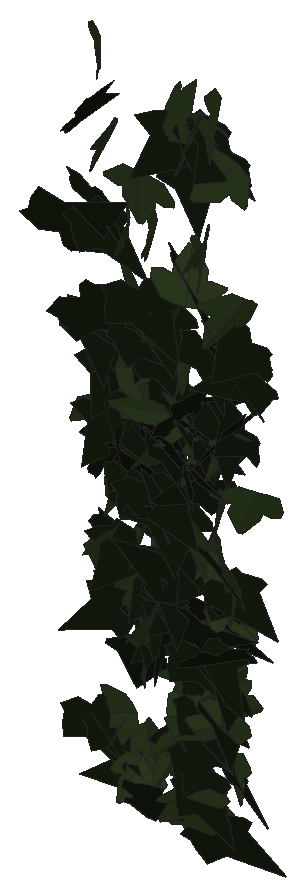
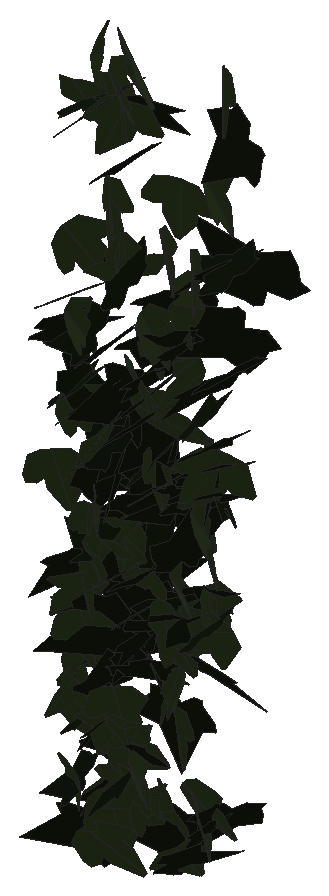
# SketchUp Ruby script. Lengths in inches.
U = 1.inch
M = Sketchup.active_model
def pt(a) = Geom::Point3d.new(a.map { |v| v * U })
def face(e, loops, mat)
  f = e.add_face(loops[0].map { |a| pt(a) })
  loops[1..].each { |l| e.add_face(l.map { |a| pt(a) }).erase! }
  f.material = f.back_material = mat if mat
  f
end
# faces: each face lists its corners as indices into pts; further lists are holes
def faces(e, pts, list, mat = nil) = list.each { |f| face(e, (f[0].is_a?(Array) ? f : [f]).map { |l| l.map { |i| pts[i] } }, mat) }
# xy, xz, yz: faces in a plane at the given z, y or x. An outline is a flat list of corners, or four numbers for a rectangle; further outlines are holes
def ring(l) = l.size == 4 ? [[l[0], l[1]], [l[2], l[1]], [l[2], l[3]], [l[0], l[3]]] : l.each_slice(2).to_a
def flat(e, list, mat, &to3) = list.each { |f| face(e, (f[0].is_a?(Array) ? f : [f]).map { |l| ring(l).map { |u, v| to3.(u, v) } }, mat) }
def xy(e, z, list, mat = nil) = flat(e, list, mat) { |x, y| [x, y, z] }
def xz(e, y, list, mat = nil) = flat(e, list, mat) { |x, z| [x, y, z] }
def yz(e, x, list, mat = nil) = flat(e, list, mat) { |y, z| [x, y, z] }
def lines(e, pts, list) = list.each { |a, b| e.add_line(pt(pts[a]), pt(pts[b])) }
# prism: a flat outline (further loops are holes) pulled along v
def prism(e, loops, v, mat = nil)
  f = face(e, loops, mat); d = Geom::Vector3d.new(v.map { |x| x * U })
  f.pushpull(f.normal.samedirection?(d) ? d.length : -d.length)
end
def box(e, o, s, mat = nil) = prism(e, [[o, [o[0] + s[0], o[1], o[2]], [o[0] + s[0], o[1] + s[1], o[2]], [o[0], o[1] + s[1], o[2]]]], [0, 0, s[2]], mat)
def at(x, y, z, deg = 0) = Geom::Transformation.translation(pt([x, y, z])) * Geom::Transformation.rotation(ORIGIN, Z_AXIS, deg.degrees)
def axes(o, x, y, z) = Geom::Transformation.new([*x, 0, *y, 0, *z, 0, *pt(o).to_a, 1])
def part(name) = M.definitions.add(name)
# library, detail: a bought-in or finely detailed component or shape, given as its bounding box
def library(name, o, s) = part(name).tap { |d| box(d.entities, o, s) }
def detail(e, o, s) = box(e.add_group.entities, o, s)
def put(e, d, t, mat = nil) = e.add_instance(d, t).tap { |i| i.material = mat if mat }
def group(e, t, mat = nil) = e.add_group.tap { |g| g.transformation = t; g.material = mat if mat }.entities
root = M.entities
M.materials.add("1026 AP 7946 SUNNY SIDE UP").color = [254, 231, 186]
M.materials.add("efeu1").color = [18, 25, 13]
M.materials.add("efeu2").color = [43, 57, 29]
c1 = part("ivyleaf_9")
p = [[1.54,2.16,1.25],[1.36,2.04,1.19],[-0.21,0.99,0.68],[-0.71,1.11,0.82],[-0.85,0.86,0.67],[-0.8,0.17,0.21],
  [-0.9,-0.01,0.1],[-0.67,-0.16,-0.02],[-0.08,-0.08,-0.05],[-0.03,-0.6,-0.4],[0.65,-0.88,-0.66],[0.83,-0.6,-0.49],
  [1.29,-0.42,-0.43],[1.8125,-0.07,-0.26],[1.21,0.44,0.15]]
faces(c1.entities,p,[[0,1,2,3,4,5,6,7,8,9,10,11,12,13,14]],"efeu1")
c2 = part("ivyleaf_10")
p = [[0,0.5,-0.03],[-0.0625,2.02,-0.43],[-0.19,2.01,-0.46],[-0.54,1.05,-0.29],[-0.52,0.625,-0.18],[-0.83,0.76,-0.28],
  [-1.16,0.64,-0.33],[-1.15,0.33,-0.24],[-0.77,-0.39,0.02],[-0.3,-0.51,0.16],[0.04,-0.48,0.23],[-0.02,2.01,-0.4375],
  [-0.06,2.01,-0.43],[0.04,-0.49,0.23],[0.67,-0.49,0.14],[1.38,0.36,-0.2],[1.375,0.51,-0.24],[0.81,0.65,-0.19],
  [0.62,0.59,-0.15],[0.6,1.09,-0.28],[0.5,1.23,-0.31]]
faces(c2.entities,p,[[0,1,2,3,4,5,6,7,8,9,10],[11,12,0,13,14,15,16,17,18,19,20]],"efeu2")
put(root,c1,axes([117.52,211.875,268.23],[0.28648,-0.02608,0.1912],[0.27976,-0.05796,-0.18851],[0.09338,0.25365,-0.02184]),"1026 AP 7946 SUNNY SIDE UP")
put(root,c1,axes([118.6,211.94,270.82],[-0.08654,-0.21141,-0.20254],[0.21087,0.15721,-0.21321],[0.40055,-0.12843,0.06849]),"1026 AP 7946 SUNNY SIDE UP")
put(root,c1,axes([117.72,211.9,273.08],[-0.07875,-0.17474,-0.24605],[0.23192,0.19414,-0.17779],[0.40196,-0.14625,0.05438]),"1026 AP 7946 SUNNY SIDE UP")
put(root,c2,axes([119.08,212.06,276.28],[-0.13153,-0.27257,0.17705],[-0.05511,-0.17041,-0.29436],[0.50497,-0.0896,0.01399]),"1026 AP 7946 SUNNY SIDE UP")
put(root,c2,axes([117.7,211.89,271.03],[-0.0112,-0.26761,-0.07503],[0.00368,0.07127,-0.27538],[0.43547,-0.00748,0.0004]),"1026 AP 7946 SUNNY SIDE UP")
put(root,c2,axes([118.51,211.85,268.5],[-0.29752,-0.20811,-0.14144],[0.16198,0.09007,-0.28887],[0.35588,-0.21498,0.01323]),"1026 AP 7946 SUNNY SIDE UP")
put(root,c1,axes([116.69,211.76,275.6875],[0.03013,-0.02962,-0.34453],[0.15877,0.3198,-0.02136],[0.5032,-0.09913,0.02737]),"1026 AP 7946 SUNNY SIDE UP")
put(root,c1,axes([117.96,212.06,272.84],[-0.19862,-0.27787,-0.08333],[0.08221,0.06315,-0.31335],[0.44687,-0.13512,0.02061]),"1026 AP 7946 SUNNY SIDE UP")
put(root,c1,axes([118.24,212,271.67],[0.00948,0.04839,0.31377],[-0.48449,0.00155,0.00605],[-0.00096,-0.30436,0.0481]),"1026 AP 7946 SUNNY SIDE UP")
put(root,c1,axes([116.18,211.92,276.53],[-0.13806,-0.01129,0.33737],[0.48746,-0.11289,0.08094],[0.16722,0.31977,0.04259]),"1026 AP 7946 SUNNY SIDE UP")
put(root,c2,axes([118.93,212.09,269.78],[-0.20767,-0.06365,0.28664],[-0.29176,-0.21433,-0.14231],[0.34176,-0.22165,0.05268]),"1026 AP 7946 SUNNY SIDE UP")
put(root,c1,axes([117.46,211.98,275.97],[-0.02587,-0.26376,-0.1741],[0.10174,0.16122,-0.26714],[0.48064,-0.04832,0.04718]),"1026 AP 7946 SUNNY SIDE UP")
put(root,c1,axes([118.86,212.17,270.36],[-0.0215,-0.24184,0.17579],[0.0172,-0.17249,-0.24995],[0.46634,-0.00479,0.01732]),"1026 AP 7946 SUNNY SIDE UP")
put(root,c1,axes([118.89,211.88,270.89],[0.12617,0.2547,-0.10383],[-0.04706,-0.09776,-0.27568],[-0.42898,0.08564,-0.0003]),"1026 AP 7946 SUNNY SIDE UP")
put(root,c2,axes([118.96,212,278.375],[0.44637,-0.10107,-0.13025],[-0.19853,0.01961,-0.30949],[0.15814,0.30991,-0.02088]),"1026 AP 7946 SUNNY SIDE UP")
put(root,c1,axes([117.26,212.15,271.91],[-0.33413,-0.16986,0.05394],[-0.03804,-0.05472,-0.27919],[0.27735,-0.21215,0.0267]),"1026 AP 7946 SUNNY SIDE UP")
put(root,c1,axes([116.59,212.13,275.25],[-0.03091,-0.30639,0.00877],[0.00098,-0.01032,-0.31635],[0.48204,-0.01962,0.0012]),"1026 AP 7946 SUNNY SIDE UP")
put(root,c2,axes([118.21,212.16,269.37],[-0.04618,-0.13865,0.24732],[-0.08507,-0.23471,-0.14736],[0.42863,-0.06152,-0.0026]),"1026 AP 7946 SUNNY SIDE UP")
put(root,c1,axes([116.9375,212.21,273.73],[-0.25318,-0.22273,0.11503],[-0.05354,-0.11352,-0.28136],[0.38899,-0.16059,0.03614]),"1026 AP 7946 SUNNY SIDE UP")
put(root,c1,axes([118.39,212.11,269.33],[-0.34798,-0.14672,-0.09231],[0.13874,0.02685,-0.27217],[0.23121,-0.23693,0.02439]),"1026 AP 7946 SUNNY SIDE UP")
put(root,c2,axes([118.3,212.15,278.79],[0.22937,-0.27854,0.1573],[0.08179,-0.14656,-0.32415],[0.49394,0.15362,-0.01937]),"1026 AP 7946 SUNNY SIDE UP")
put(root,c1,axes([118.48,211.99,268.75],[0.10046,-0.25601,-0.17354],[-0.07577,0.16004,-0.2708],[0.47461,0.07974,-0.0065]),"1026 AP 7946 SUNNY SIDE UP")
put(root,c2,axes([119.02,211.91,272.3],[-0.29534,0.16954,0.13274],[-0.16581,0.07374,-0.25983],[-0.28985,-0.21493,0.01338]),"1026 AP 7946 SUNNY SIDE UP")
put(root,c1,axes([119.06,212.16,274.43],[-0.22278,0.08039,-0.25038],[0.18537,-0.22663,-0.14907],[-0.35806,-0.16734,0.07861]),"1026 AP 7946 SUNNY SIDE UP")
put(root,c2,axes([118.93,212.23,270.49],[-0.02652,-0.09055,0.28616],[0.03241,-0.27843,-0.09367],[0.45902,0.01443,0.02315]),"1026 AP 7946 SUNNY SIDE UP")
put(root,c1,axes([118.61,212.18,272.15],[0.09758,-0.21951,0.17614],[0.13105,-0.1538,-0.23377],[0.41869,0.0993,0.03212]),"1026 AP 7946 SUNNY SIDE UP")
put(root,c1,axes([117.9,212.19,271.45],[-0.03382,-0.27615,0.06888],[0.00761,-0.06897,-0.28557],[0.44729,-0.01971,0.01007]),"1026 AP 7946 SUNNY SIDE UP")
put(root,c1,axes([117.03,211.79,273.34],[-0.01053,0.15468,0.27091],[-0.04215,0.26084,-0.15777],[-0.47668,-0.02648,0.00796]),"1026 AP 7946 SUNNY SIDE UP")
put(root,c1,axes([118.1875,212.19,278.5625],[-0.43637,-0.12441,0.05251],[-0.05425,-0.04876,-0.31208],[0.20477,-0.27805,0.02923]),"1026 AP 7946 SUNNY SIDE UP")
put(root,c1,axes([117.09,212.09,270.95],[-0.4232,0.05156,0.02258],[-0.04237,-0.02643,-0.28066],[-0.07703,-0.26872,0.03029]),"1026 AP 7946 SUNNY SIDE UP")
put(root,c2,axes([118.57,212.25,279.1],[0.04692,-0.13884,0.30306],[0.27055,-0.24488,-0.13811],[0.43541,0.16712,0.05316]),"1026 AP 7946 SUNNY SIDE UP")
put(root,c1,axes([117.01,212.01,273.27],[0.49346,-0.07383,0.08195],[0.11295,-0.04286,-0.33142],[0.12858,0.32101,-0.02338]),"1026 AP 7946 SUNNY SIDE UP")
put(root,c1,axes([116.99,211.9375,273.8125],[0.27214,-0.11016,-0.28023],[-0.39822,0.10206,-0.20847],[0.23135,0.30527,-0.02921]),"1026 AP 7946 SUNNY SIDE UP")
put(root,c2,axes([117.93,212.04,274.25],[0.15627,-0.02437,-0.31235],[-0.46878,0.05472,-0.10493],[0.09376,0.31421,-0.00405]),"1026 AP 7946 SUNNY SIDE UP")
put(root,c2,axes([117.9375,212.12,278.8],[0.32996,-0.27339,-0.11813],[0.12994,-0.079,0.35417],[-0.44671,-0.22492,0.01577]),"1026 AP 7946 SUNNY SIDE UP")
put(root,c2,axes([116.85,212.09,271.9375],[-0.01041,-0.29144,-0.00215],[-0.00395,0.00049,-0.3003],[0.45824,-0.00661,-0.00264]),"1026 AP 7946 SUNNY SIDE UP")
put(root,c1,axes([117.69,212.15,273.58],[0.31328,-0.16327,0.20022],[0.22087,-0.13629,-0.26582],[0.33378,0.24342,-0.01202]),"1026 AP 7946 SUNNY SIDE UP")
put(root,c1,axes([118.69,212.27,269.74],[0.01946,-0.25785,0.14319],[0.03169,-0.13951,-0.26648],[0.4606,0.02049,0.01228]),"1026 AP 7946 SUNNY SIDE UP")
put(root,c1,axes([117.72,212.2,271.25],[0.03628,-0.09601,0.34374],[0.36991,-0.24235,-0.08987],[0.40265,0.23129,0.0516]),"1026 AP 7946 SUNNY SIDE UP")
put(root,c2,axes([118.54,211.98,277.09],[0.02059,-0.26895,-0.17339],[-0.01235,0.16659,-0.27642],[0.49745,0.01527,0.00031]),"1026 AP 7946 SUNNY SIDE UP")
put(root,c2,axes([118.98,212.23,274.02],[-0.05505,-0.21615,0.18845],[-0.0449,-0.18193,-0.22664],[0.44424,-0.04517,0.00044]),"1026 AP 7946 SUNNY SIDE UP")
put(root,c2,axes([118.41,212.14,268.53],[-0.23096,-0.30836,0.04221],[-0.00826,-0.04478,-0.35182],[0.48943,-0.14627,0.01398]),"1026 AP 7946 SUNNY SIDE UP")
put(root,c1,axes([118.97,212.34,274.22],[-0.15595,-0.16039,0.23349],[-0.05027,-0.23341,-0.1852],[0.43486,-0.0845,0.06233]),"1026 AP 7946 SUNNY SIDE UP")
put(root,c1,axes([118.54,212.28,273.3125],[-0.09857,-0.01054,-0.29561],[0.00897,-0.29364,0.00811],[-0.45132,-0.00353,0.06472]),"1026 AP 7946 SUNNY SIDE UP")
put(root,c1,axes([117.73,212.23,270.82],[-0.21036,0.01814,-0.24938],[0.34706,-0.10626,-0.13443],[-0.1593,-0.25546,0.03645]),"1026 AP 7946 SUNNY SIDE UP")
put(root,c1,axes([118.6875,212.37,278.41],[-0.2355,-0.1882,0.2191],[-0.0148,-0.2381,-0.22416],[0.44757,-0.1069,0.10788]),"1026 AP 7946 SUNNY SIDE UP")
put(root,c1,axes([117.69,212.21,273.67],[0.16616,-0.27745,0.0239],[-0.00034,-0.02658,-0.30585],[0.438,0.10523,-0.00931]),"1026 AP 7946 SUNNY SIDE UP")
put(root,c2,axes([118.13,212.14,272.5],[-0.35983,0.15957,-0.12434],[0.13006,-0.09301,-0.28664],[-0.28739,-0.24187,0.02596]),"1026 AP 7946 SUNNY SIDE UP")
put(root,c1,axes([116.57,212.1,276.82],[0.16705,-0.25483,-0.16262],[0.02024,0.16973,-0.27488],[0.46971,0.08331,0.06968]),"1026 AP 7946 SUNNY SIDE UP")
put(root,c2,axes([118.42,212.2,272.12],[-0.36616,0.06865,0.15527],[-0.25413,-0.14885,-0.18875],[0.05427,-0.23381,0.16372]),"1026 AP 7946 SUNNY SIDE UP")
put(root,c1,axes([119.04,212.38,275.5625],[-0.23934,-0.20927,0.17215],[-0.03837,-0.18187,-0.25678],[0.42052,-0.1357,0.07455]),"1026 AP 7946 SUNNY SIDE UP")
put(root,c1,axes([118.34,212.17,269.79],[0.11619,-0.26871,-0.10711],[-0.02996,0.10097,-0.28639],[0.45119,0.0759,0.00857]),"1026 AP 7946 SUNNY SIDE UP")
put(root,c2,axes([117.71,212.13,273.63],[-0.04387,-0.28618,-0.05682],[-0.0038,0.054,-0.29581],[0.45778,-0.02698,-0.0079]),"1026 AP 7946 SUNNY SIDE UP")
put(root,c2,axes([117.35,211.89,274.8],[-0.03685,0.12198,0.32859],[-0.08308,0.31386,-0.12609],[-0.52946,-0.05774,-0.00308]),"1026 AP 7946 SUNNY SIDE UP")
put(root,c1,axes([116.83,212.13,275.03],[0.12815,-0.25021,-0.1735],[-0.00672,0.17203,-0.26668],[0.47296,0.07024,0.04322]),"1026 AP 7946 SUNNY SIDE UP")
put(root,c2,axes([117.26,212.29,272.11],[0.21592,-0.20647,0.15372],[0.10698,-0.135,-0.25574],[0.38712,0.15247,-0.01506]),"1026 AP 7946 SUNNY SIDE UP")
put(root,c2,axes([118.77,212.07,273.01],[0.14368,-0.28317,-0.16915],[-0.03618,0.16282,-0.30453],[0.51215,0.09095,0.02594]),"1026 AP 7946 SUNNY SIDE UP")
put(root,c1,axes([116.51,211.87,278.46],[0.11623,0.21715,0.25415],[0.16315,0.22319,-0.23428],[-0.48882,0.12612,-0.01776]),"1026 AP 7946 SUNNY SIDE UP")
put(root,c2,axes([117.35,212.16,277.58],[-0.47703,0.0082,0.02049],[-0.03312,-0.05937,-0.30687],[-0.00652,-0.29817,0.05985]),"1026 AP 7946 SUNNY SIDE UP")
put(root,c1,axes([117.47,212.37,273.43],[-0.07248,-0.29275,0.10869],[0.00608,-0.10886,-0.30528],[0.49016,-0.04194,0.01986]),"1026 AP 7946 SUNNY SIDE UP")
put(root,c1,axes([118.67,212.34,274.1875],[-0.01813,-0.28718,0.07632],[-0.00848,-0.07555,-0.29652],[0.46692,-0.01252,-0.00242]),"1026 AP 7946 SUNNY SIDE UP")
put(root,c1,axes([119.24,212.38,275.0625],[-0.24661,-0.0948,0.24494],[-0.26373,-0.1734,-0.18579],[0.30506,-0.22653,0.03738]),"1026 AP 7946 SUNNY SIDE UP")
put(root,c2,axes([118.43,212.08,276.82],[0.22358,-0.24187,-0.15999],[-0.03153,0.16301,-0.28201],[0.4497,0.13168,0.05977]),"1026 AP 7946 SUNNY SIDE UP")
put(root,c1,axes([118.12,212.18,270.87],[0.1079,-0.0622,0.27328],[0.38926,-0.10089,-0.09081],[0.18025,0.25512,0.03253]),"1026 AP 7946 SUNNY SIDE UP")
put(root,c1,axes([117.25,212.0625,275.38],[0.19287,-0.17061,-0.23498],[-0.07321,0.23198,-0.20406],[0.44063,0.11322,0.06895]),"1026 AP 7946 SUNNY SIDE UP")
put(root,c1,axes([118.64,212.1,268.05],[0.03797,-0.04282,-0.29382],[0.29719,0.21822,-0.016],[0.34204,-0.18485,0.04652]),"1026 AP 7946 SUNNY SIDE UP")
put(root,c1,axes([117.86,212.05,273.98],[0.4215,0.13599,0.0126],[0.03419,-0.01764,-0.30864],[-0.21185,0.26772,-0.02475]),"1026 AP 7946 SUNNY SIDE UP")
put(root,c2,axes([117.76,212.37,268.78],[-0.04315,-0.16404,0.22454],[0.08245,-0.21906,-0.16364],[0.42213,0.02602,0.05491]),"1026 AP 7946 SUNNY SIDE UP")
put(root,c2,axes([117.47,212,275.87],[-0.13702,0.14631,-0.32569],[-0.27612,0.26399,0.17681],[0.47444,0.19589,0.00884]),"1026 AP 7946 SUNNY SIDE UP")
put(root,c1,axes([117.77,212.3,274.5625],[0.08597,-0.28877,-0.01771],[-0.02427,0.01289,-0.30241],[0.45407,0.05536,-0.01281]),"1026 AP 7946 SUNNY SIDE UP")
put(root,c1,axes([118.25,212.43,271.86],[-0.16686,-0.20642,0.17179],[-0.04591,-0.17066,-0.23612],[0.41588,-0.10166,0.04286]),"1026 AP 7946 SUNNY SIDE UP")
put(root,c1,axes([116.49,212.2,269.11],[-0.02007,-0.22965,-0.17641],[0.02554,0.16924,-0.23589],[0.44848,-0.01992,0.00554]),"1026 AP 7946 SUNNY SIDE UP")
put(root,c2,axes([117.31,212.31,271.36],[-0.05303,-0.27545,0.11092],[-0.00206,-0.1098,-0.2863],[0.46593,-0.03184,0.01136]),"1026 AP 7946 SUNNY SIDE UP")
put(root,c2,axes([117.76,212.23,275.52],[-0.00279,-0.29758,-0.00929],[-0.01574,0.00738,-0.30636],[0.4678,-0.00153,-0.01037]),"1026 AP 7946 SUNNY SIDE UP")
put(root,c1,axes([117.35,212.41,270.74],[-0.04108,-0.25177,0.12532],[-0.0207,-0.12237,-0.26148],[0.44016,-0.02925,-0.0006]),"1026 AP 7946 SUNNY SIDE UP")
put(root,c1,axes([116.79,212.45,274.6],[-0.0635,-0.20606,0.22246],[-0.00907,-0.2185,-0.21602],[0.47058,-0.03201,0.02585]),"1026 AP 7946 SUNNY SIDE UP")
put(root,c1,axes([116.94,212.38,273.41],[-0.20535,-0.2531,0.02817],[-0.00298,-0.03138,-0.2933],[0.40053,-0.13,0.01226]),"1026 AP 7946 SUNNY SIDE UP")
put(root,c1,axes([117.46,212.42,272.57],[0.06045,-0.19064,0.21887],[0.03774,-0.21255,-0.20119],[0.44853,0.04358,-0.01257]),"1026 AP 7946 SUNNY SIDE UP")
put(root,c2,axes([118.42,212.32,273.76],[0.17194,0.19573,-0.18475],[-0.16373,-0.14808,-0.23136],[-0.38525,0.15029,0.01587]),"1026 AP 7946 SUNNY SIDE UP")
put(root,c1,axes([117.61,212.39,271.49],[-0.30105,-0.19453,0.04776],[-0.02912,-0.04819,-0.28069],[0.3135,-0.19128,0.0198]),"1026 AP 7946 SUNNY SIDE UP")
put(root,c1,axes([117.31,212.16,270.3],[0.32008,0.06624,-0.17792],[-0.24788,-0.07327,-0.22032],[-0.1532,0.25695,-0.01524]),"1026 AP 7946 SUNNY SIDE UP")
put(root,c1,axes([117.77,212.36,273.2],[-0.1637,-0.29448,-0.04317],[0.02187,0.03775,-0.32155],[0.46684,-0.10503,-0.00007]),"1026 AP 7946 SUNNY SIDE UP")
put(root,c2,axes([118.4375,212.17,278.7],[0.30452,-0.2024,-0.1354],[-0.0983,0.11918,-0.28579],[0.3655,0.20069,0.03595]),"1026 AP 7946 SUNNY SIDE UP")
put(root,c1,axes([118.875,212.16,271.85],[0.05079,-0.18184,-0.22487],[0.02339,0.21944,-0.18566],[0.44486,0.00923,0.03543]),"1026 AP 7946 SUNNY SIDE UP")
put(root,c2,axes([118.17,212.11,276.17],[0.32805,0.2315,-0.08393],[0.06168,0.07584,0.32077],[0.38164,-0.21125,0.02031]),"1026 AP 7946 SUNNY SIDE UP")
put(root,c1,axes([117.11,212.33,271.62],[0.24537,-0.17169,0.17302],[0.17553,-0.12681,-0.23975],[0.3356,0.19186,-0.00111]),"1026 AP 7946 SUNNY SIDE UP")
put(root,c2,axes([117.92,212.29,274.82],[0.312,-0.21718,0.02197],[-0.00362,-0.03256,-0.30227],[0.34331,0.19703,-0.02315]),"1026 AP 7946 SUNNY SIDE UP")
put(root,c1,axes([117.92,212.47,276.1875],[0.11923,-0.23926,0.2441],[0.0719,-0.23471,-0.25913],[0.52609,0.0863,-0.01991]),"1026 AP 7946 SUNNY SIDE UP")
put(root,c2,axes([117.23,212.3,271.41],[-0.39015,-0.09258,-0.16764],[-0.25654,-0.02383,0.27098],[-0.14293,0.29548,-0.02877]),"1026 AP 7946 SUNNY SIDE UP")
put(root,c1,axes([117.58,212.28,274.99],[0.07311,-0.27265,-0.10808],[0.00478,0.10512,-0.28362],[0.45846,0.04238,0.02019]),"1026 AP 7946 SUNNY SIDE UP")
put(root,c1,axes([118.13,211.95,274.33],[-0.03431,0.16741,-0.30416],[-0.10014,0.28955,0.17512],[0.52553,0.0661,0.01351]),"1026 AP 7946 SUNNY SIDE UP")
put(root,c1,axes([117.86,212.42,270.77],[-0.33818,-0.15261,0.08271],[-0.07643,-0.07091,-0.27051],[0.26081,-0.21866,0.02797]),"1026 AP 7946 SUNNY SIDE UP")
put(root,c1,axes([118.01,212.41,277.875],[-0.00994,-0.30328,0.03774],[0.00237,-0.0384,-0.31272],[0.48068,-0.00608,0.00232]),"1026 AP 7946 SUNNY SIDE UP")
put(root,c2,axes([117.25,212.37,268.91],[0.23211,-0.0617,0.22351],[0.29259,-0.11397,-0.16422],[0.2014,0.23669,-0.01901]),"1026 AP 7946 SUNNY SIDE UP")
put(root,c1,axes([117.25,212.5,275.09],[-0.09415,-0.26466,0.17214],[-0.02779,-0.16852,-0.27998],[0.49263,-0.06008,0.0171]),"1026 AP 7946 SUNNY SIDE UP")
put(root,c1,axes([118.18,212.45,273.75],[0.09401,-0.18944,0.23962],[0.12786,-0.2192,-0.20579],[0.4554,0.10065,0.00831]),"1026 AP 7946 SUNNY SIDE UP")
put(root,c1,axes([116.6875,212.49,274.29],[-0.17676,-0.23539,0.13262],[-0.03583,-0.13214,-0.26741],[0.42136,-0.10998,0.0329]),"1026 AP 7946 SUNNY SIDE UP")
put(root,c2,axes([117.67,212.36,272.16],[0.28834,-0.05317,0.22646],[0.32927,-0.06802,-0.19703],[0.13556,0.27831,-0.00311]),"1026 AP 7946 SUNNY SIDE UP")
put(root,c1,axes([118.54,212.37,275.22],[0.27744,-0.23133,0.06104],[0.03656,-0.05831,-0.29958],[0.37422,0.1772,-0.01599]),"1026 AP 7946 SUNNY SIDE UP")
put(root,c2,axes([117.15,212.37,268.38],[0.22385,0.18172,-0.14127],[-0.10281,-0.12354,-0.23753],[-0.3439,0.15522,-0.02094]),"1026 AP 7946 SUNNY SIDE UP")
put(root,c2,axes([116.64,212.28,271.62],[-0.25117,0.00983,-0.25818],[0.3872,-0.05061,-0.16399],[-0.07534,-0.2929,0.01791]),"1026 AP 7946 SUNNY SIDE UP")
put(root,c1,axes([118.5,212.18,270.21],[-0.263,-0.14182,0.20693],[0.21023,0.15258,0.22567],[-0.32572,0.213,-0.02143]),"1026 AP 7946 SUNNY SIDE UP")
put(root,c2,axes([116.68,212.21,273.9375],[-0.34414,-0.19028,-0.17142],[0.22914,0.08313,-0.29683],[0.3234,-0.26138,0.0279]),"1026 AP 7946 SUNNY SIDE UP")
put(root,c1,axes([118.27,212.25,278.66],[0.23597,-0.26231,-0.16089],[-0.03576,0.16232,-0.30534],[0.4775,0.14178,0.05665]),"1026 AP 7946 SUNNY SIDE UP")
put(root,c2,axes([118.01,212.3,269.02],[-0.36954,0.06419,-0.12666],[0.16475,-0.07741,-0.24768],[-0.14367,-0.25387,0.04178]),"1026 AP 7946 SUNNY SIDE UP")
put(root,c1,axes([117.75,212.24,271.14],[0.05442,-0.20215,-0.19228],[-0.0673,0.1807,-0.21004],[0.42612,0.05436,-0.00862]),"1026 AP 7946 SUNNY SIDE UP")
put(root,c2,axes([118.4,212.43,272.16],[0.1192,-0.07645,0.27431],[0.3567,-0.1421,-0.10922],[0.25117,0.23809,0.02493]),"1026 AP 7946 SUNNY SIDE UP")
put(root,c2,axes([118.22,212.32,270.15],[-0.34234,-0.16367,0.06087],[-0.0507,-0.05655,-0.27972],[0.26938,-0.21864,0.0247]),"1026 AP 7946 SUNNY SIDE UP")
put(root,c2,axes([118.78,212.18,271.52],[0.14931,0.21937,0.15561],[0.12575,0.1281,-0.24472],[-0.39831,0.12267,-0.01893]),"1026 AP 7946 SUNNY SIDE UP")
put(root,c1,axes([118.19,212.17,273.54],[0.15405,-0.1047,-0.25946],[-0.3006,0.16363,-0.14608],[0.30468,0.21437,-0.01293]),"1026 AP 7946 SUNNY SIDE UP")
put(root,c2,axes([118.84,212.18,271.72],[0.22961,-0.16423,-0.20356],[-0.11021,0.19212,-0.21777],[0.38751,0.15195,0.05868]),"1026 AP 7946 SUNNY SIDE UP")
put(root,c2,axes([117.45,212.28,276.85],[0.16357,-0.27734,-0.06729],[0.00105,0.06811,-0.30375],[0.44747,0.10122,0.02531]),"1026 AP 7946 SUNNY SIDE UP")
put(root,c2,axes([116.8,212.4375,273.21],[0.12436,-0.23148,0.15914],[0.09039,-0.14493,-0.25277],[0.42932,0.09757,0.00712]),"1026 AP 7946 SUNNY SIDE UP")
put(root,c2,axes([116.55,212.21,279.4375],[0.23927,-0.24308,-0.14546],[0.01131,0.16241,-0.28186],[0.44079,0.12778,0.08619]),"1026 AP 7946 SUNNY SIDE UP")
put(root,c1,axes([117.22,212.48,268.22],[-0.22451,-0.05661,0.2365],[-0.26986,-0.16019,-0.15138],[0.25646,-0.21812,0.04775]),"1026 AP 7946 SUNNY SIDE UP")
put(root,c1,axes([116.64,212.29,268.92],[0.1113,-0.21335,-0.14],[-0.03886,0.13335,-0.23021],[0.39482,0.07327,0.01681]),"1026 AP 7946 SUNNY SIDE UP")
put(root,c2,axes([117.63,212.4,275.69],[0.04617,-0.28567,0.0873],[0.00507,-0.08647,-0.2963],[0.46924,0.02904,-0.00539]),"1026 AP 7946 SUNNY SIDE UP")
put(root,c1,axes([117.45,212.39,275.57],[-0.10884,-0.2746,-0.10673],[0.06589,0.0945,-0.29069],[0.45589,-0.07922,0.01653]),"1026 AP 7946 SUNNY SIDE UP")
put(root,c2,axes([117.25,212.28,270.71],[-0.22677,0.24883,-0.02655],[0.00054,-0.03117,-0.29605],[-0.39358,-0.14341,0.01489]),"1026 AP 7946 SUNNY SIDE UP")
put(root,c1,axes([116.25,212.48,276.92],[0.09684,-0.25846,0.14506],[0.12552,-0.12532,-0.27087],[0.44661,0.09127,0.04467]),"1026 AP 7946 SUNNY SIDE UP")
put(root,c2,axes([117.875,212.36,269.27],[0.1498,-0.25964,0.00967],[-0.00601,-0.01297,-0.28488],[0.40858,0.09501,-0.00774]),"1026 AP 7946 SUNNY SIDE UP")
put(root,c2,axes([116.99,212.26,269.2],[0.20195,-0.11658,-0.23738],[-0.30606,0.1243,-0.17633],[0.26542,0.23203,-0.02272]),"1026 AP 7946 SUNNY SIDE UP")
put(root,c1,axes([118.24,212.44,275.22],[0.05686,-0.29293,-0.00474],[-0.01145,0.00206,-0.30397],[0.46049,0.03622,-0.00697]),"1026 AP 7946 SUNNY SIDE UP")
put(root,c1,axes([117.16,212.33,272.51],[0.11825,0.20428,0.18676],[-0.32104,-0.08139,0.18242],[0.28342,-0.17742,0.12872]),"1026 AP 7946 SUNNY SIDE UP")
put(root,c1,axes([117.73,212.52,272.12],[-0.14957,-0.2552,0.08683],[-0.00942,-0.0889,-0.27998],[0.42321,-0.09217,0.02445]),"1026 AP 7946 SUNNY SIDE UP")
put(root,c2,axes([119.15,212.36,273.2],[-0.35834,-0.16353,0.07683],[-0.07709,-0.06085,-0.28857],[0.27252,-0.23224,0.01939]),"1026 AP 7946 SUNNY SIDE UP")
put(root,c2,axes([116.91,212.29,269.01],[0.107,-0.25826,-0.10128],[-0.05216,0.09136,-0.27447],[0.43055,0.07525,-0.00808]),"1026 AP 7946 SUNNY SIDE UP")
put(root,c1,axes([118.23,212.24,271.12],[0.45853,0.03233,0.10829],[0.16899,-0.02307,-0.3005],[-0.03535,0.30905,-0.03192]),"1026 AP 7946 SUNNY SIDE UP")
put(root,c1,axes([116.65,212.55,271.67],[-0.03467,-0.23067,0.18903],[0.01531,-0.18578,-0.23879],[0.4645,-0.01109,0.02198]),"1026 AP 7946 SUNNY SIDE UP")
put(root,c2,axes([118.46,212.41,268.13],[-0.22731,-0.06368,0.23358],[-0.29631,-0.129,-0.16159],[0.22302,-0.23629,0.02338]),"1026 AP 7946 SUNNY SIDE UP")
put(root,c2,axes([116.87,212.16,272.67],[0.046,-0.09973,-0.27955],[-0.15654,0.25198,-0.10521],[0.4259,0.10339,-0.00848]),"1026 AP 7946 SUNNY SIDE UP")
put(root,c2,axes([118.14,212.3,269.78],[0.33286,0.15144,0.10277],[0.14174,0.04366,-0.26739],[-0.24657,0.22954,-0.01497]),"1026 AP 7946 SUNNY SIDE UP")
put(root,c1,axes([118.4,212.18,273.92],[0.2459,-0.08297,-0.24593],[-0.22763,0.20006,-0.1685],[0.32488,0.20297,0.06809]),"1026 AP 7946 SUNNY SIDE UP")
put(root,c2,axes([118.7,212.36,271.08],[-0.37041,-0.11743,0.07009],[-0.07156,-0.06145,-0.26931],[0.20161,-0.23756,0.03319]),"1026 AP 7946 SUNNY SIDE UP")
put(root,c2,axes([116.58,212.43,277.98],[0.1178,-0.28764,0.06816],[0.01037,-0.0683,-0.30641],[0.46456,0.07446,-0.01044]),"1026 AP 7946 SUNNY SIDE UP")
put(root,c1,axes([118.08,212.28,269.12],[0.2929,-0.14674,-0.13817],[-0.15297,0.09169,-0.24352],[0.27159,0.20989,0.01185]),"1026 AP 7946 SUNNY SIDE UP")
put(root,c2,axes([118.09,212.3,278.53],[-0.32862,-0.19867,-0.11393],[0.17456,0.04022,-0.29331],[0.31104,-0.23247,0.04423]),"1026 AP 7946 SUNNY SIDE UP")
put(root,c2,axes([118.96,212.18,270.09],[-0.04173,-0.16381,-0.23791],[0.13218,0.21597,-0.16718],[0.42389,-0.08347,0.02871]),"1026 AP 7946 SUNNY SIDE UP")
put(root,c1,axes([118.68,212.41,268.91],[0.25123,-0.2269,0.02076],[-0.00102,-0.02664,-0.28558],[0.35837,0.15899,-0.01537]),"1026 AP 7946 SUNNY SIDE UP")
put(root,c2,axes([117,212.28,276.73],[0.11855,-0.25961,-0.13692],[0.00482,0.13647,-0.27509],[0.45751,0.06583,0.03837]),"1026 AP 7946 SUNNY SIDE UP")
put(root,c2,axes([117.24,212.28,270.17],[0.26115,-0.18104,-0.13811],[-0.04151,0.14857,-0.24136],[0.35081,0.15235,0.07425]),"1026 AP 7946 SUNNY SIDE UP")
put(root,c2,axes([118.76,212.48,268.9],[-0.20759,0.11253,-0.2004],[0.09417,-0.20054,-0.16203],[-0.34149,-0.12371,0.07714]),"1026 AP 7946 SUNNY SIDE UP")
put(root,c2,axes([117.36,212.25,270.72],[-0.1441,0.25012,0.11928],[-0.09209,0.10003,-0.27315],[-0.42253,-0.1071,0.01885]),"1026 AP 7946 SUNNY SIDE UP")
put(root,c2,axes([118.72,212.51,275.44],[0.10672,-0.24863,0.15065],[0.05537,-0.14343,-0.26632],[0.4513,0.07639,-0.00295]),"1026 AP 7946 SUNNY SIDE UP")
put(root,c1,axes([117.76,212.54,274.28],[-0.02214,-0.28899,0.05757],[-0.00636,-0.05739,-0.2984],[0.46328,-0.0146,-0.00135]),"1026 AP 7946 SUNNY SIDE UP")
